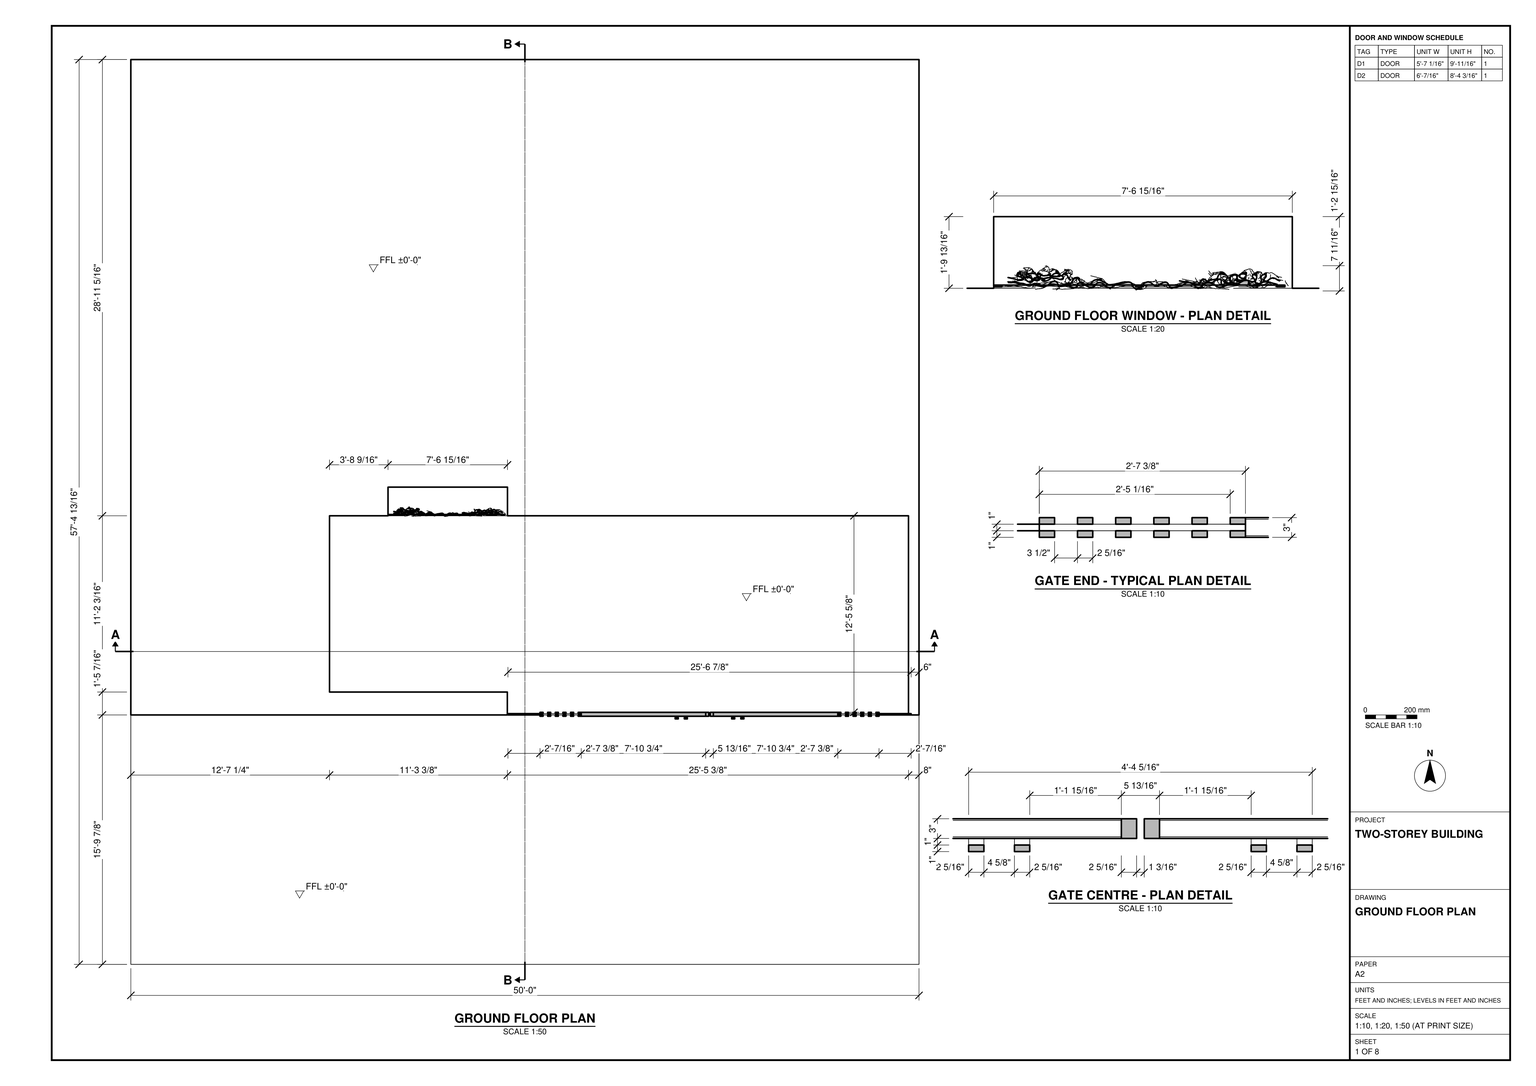
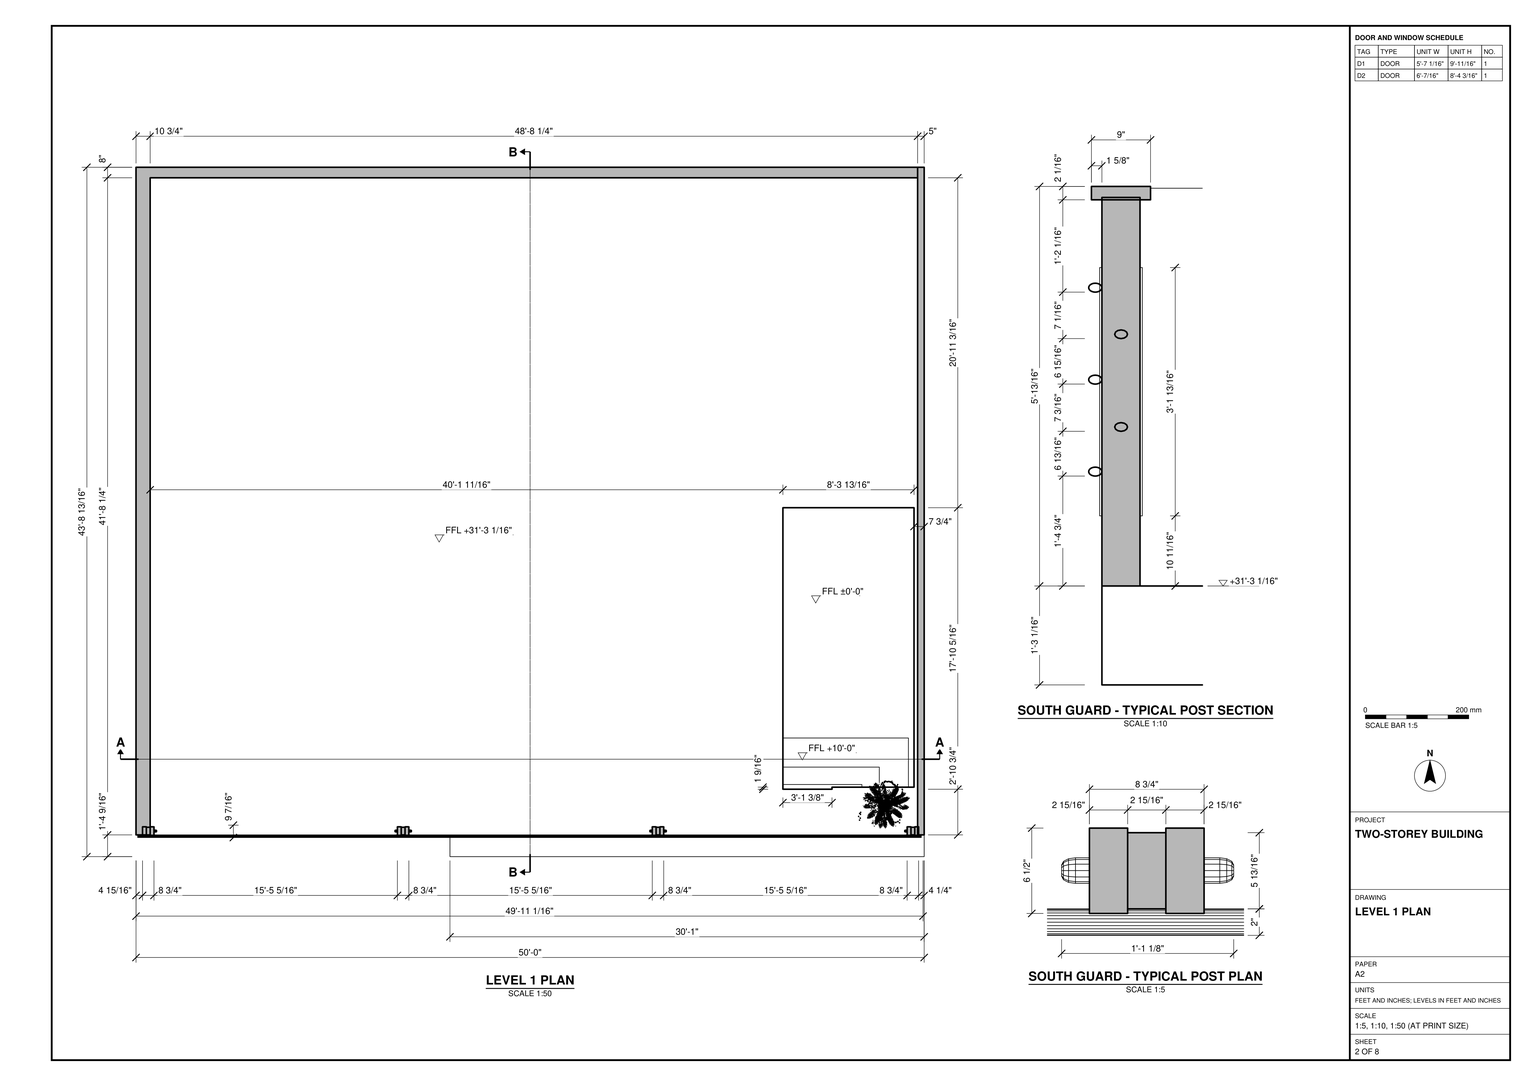
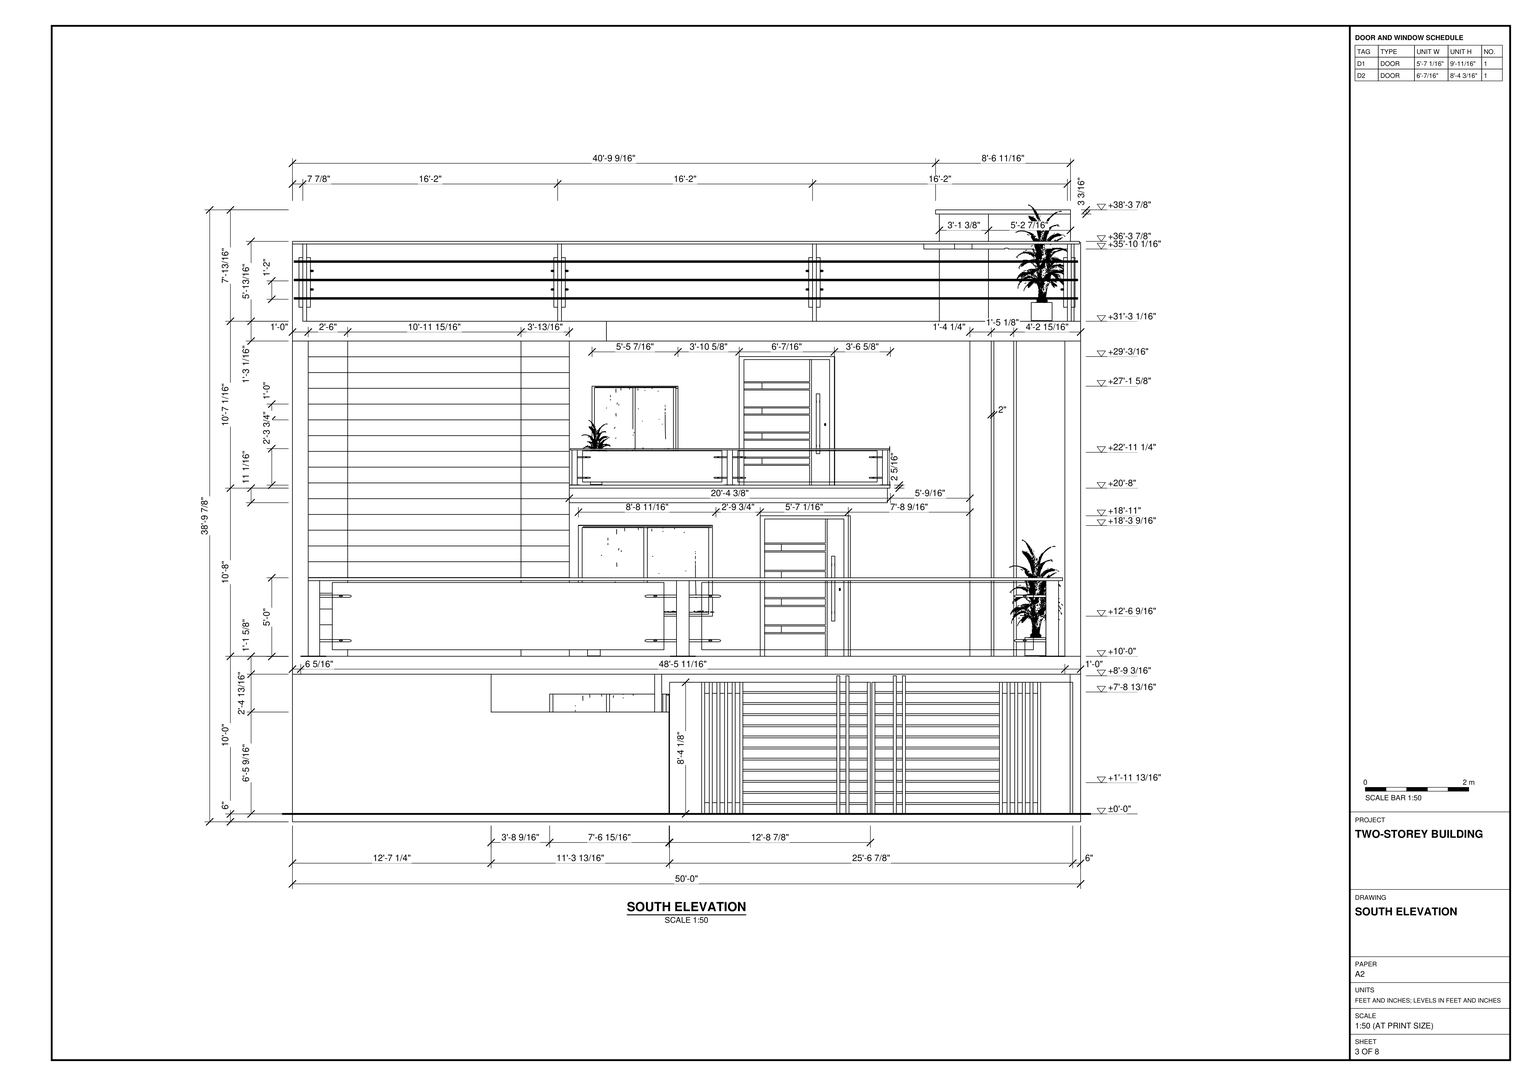
Build the two-storey building in SketchUp from task_files/diagram_01.pdf. Work in feet and inches. Set out the complete model at 50'-0" wide by 57'-4 13/16" deep, with an overall height of 39'-2 5/8". Use ±0'-0" as the ground-floor datum and +31'-3 1/16" as the upper terrace level.

Follow the plans for the ground slab, wall returns, wall thicknesses and projecting ground-floor window feature. On the south frontage, place the two-leaf gate to the right of the stepped solid wall. Use the gate details to distinguish the horizontal slats from the closely spaced vertical end members. Above the gate, model the broad lower balcony and the shorter balcony above it, including their slab edges and panel guards. Set the windows and doors behind the guards as shown in elevation, with the horizontally divided wall panel to their left. Model the flat roof terrace with its rectangular opening, perimeter walls and post-and-rail guard along the south edge.

Keep walls, slabs, roof and each furniture or joinery piece shown in separate groups or components. Use components for repeated parts such as guard posts. Decor and loose items, including plants, may be any suitable library components. Save one SketchUp model as output_files/two_storey_building_with_balconies_and_a_gated_frontage.skp.

# SketchUp Ruby script. Lengths in inches.
U = 1.inch
M = Sketchup.active_model
def pt(a) = Geom::Point3d.new(a.map { |v| v * U })
def face(e, loops, mat)
  f = e.add_face(loops[0].map { |a| pt(a) })
  loops[1..].each { |l| e.add_face(l.map { |a| pt(a) }).erase! }
  f.material = f.back_material = mat if mat
  f
end
# faces: each face lists its corners as indices into pts; further lists are holes
def faces(e, pts, list, mat = nil) = list.each { |f| face(e, (f[0].is_a?(Array) ? f : [f]).map { |l| l.map { |i| pts[i] } }, mat) }
# xy, xz, yz: faces in a plane at the given z, y or x. An outline is a flat list of corners, or four numbers for a rectangle; further outlines are holes
def ring(l) = l.size == 4 ? [[l[0], l[1]], [l[2], l[1]], [l[2], l[3]], [l[0], l[3]]] : l.each_slice(2).to_a
def flat(e, list, mat, &to3) = list.each { |f| face(e, (f[0].is_a?(Array) ? f : [f]).map { |l| ring(l).map { |u, v| to3.(u, v) } }, mat) }
def xy(e, z, list, mat = nil) = flat(e, list, mat) { |x, y| [x, y, z] }
def xz(e, y, list, mat = nil) = flat(e, list, mat) { |x, z| [x, y, z] }
def yz(e, x, list, mat = nil) = flat(e, list, mat) { |y, z| [x, y, z] }
def lines(e, pts, list) = list.each { |a, b| e.add_line(pt(pts[a]), pt(pts[b])) }
# prism: a flat outline (further loops are holes) pulled along v
def prism(e, loops, v, mat = nil)
  f = face(e, loops, mat); d = Geom::Vector3d.new(v.map { |x| x * U })
  f.pushpull(f.normal.samedirection?(d) ? d.length : -d.length)
end
def box(e, o, s, mat = nil) = prism(e, [[o, [o[0] + s[0], o[1], o[2]], [o[0] + s[0], o[1] + s[1], o[2]], [o[0], o[1] + s[1], o[2]]]], [0, 0, s[2]], mat)
def at(x, y, z, deg = 0) = Geom::Transformation.translation(pt([x, y, z])) * Geom::Transformation.rotation(ORIGIN, Z_AXIS, deg.degrees)
def axes(o, x, y, z) = Geom::Transformation.new([*x, 0, *y, 0, *z, 0, *pt(o).to_a, 1])
def part(name) = M.definitions.add(name)
# library, detail: a bought-in or finely detailed component or shape, given as its bounding box
def library(name, o, s) = part(name).tap { |d| box(d.entities, o, s) }
def detail(e, o, s) = box(e.add_group.entities, o, s)
def put(e, d, t, mat = nil) = e.add_instance(d, t).tap { |i| i.material = mat if mat }
def group(e, t, mat = nil) = e.add_group.tap { |g| g.transformation = t; g.material = mat if mat }.entities
root = M.entities
M.materials.add("EWSZ RGF 1").color = [166, 112, 73]
M.materials.add("VBGD1").color = [203, 203, 203]
M.materials.add("W4E SDT G1").color = [255, 255, 255]
M.materials.add("W4E SESF XVD1").color = [203, 203, 203]
M.materials.add("[0131_Silver]").color = [192, 192, 192]
M.materials.add("[Color M07]").color = [58, 58, 58]
M.materials.add("[Color_002]").color = [172, 198, 184]
M.materials["[Color_002]"].alpha = 0.07
M.materials.add("[Field Rectangle Tile]").color = [196, 189, 179]
M.materials.add("[Wood Veneer 01]").color = [120, 70, 37]
c1 = part("Panel mounting bracket")
xy(c1.entities,-0.08,[[2.57,0.63,2.46,0.64,2.36,0.69,2.28,0.75,2.21,0.84,2.17,0.9375,2.15,1.05,2.17,1.15,2.21,1.25,2.27,1.34,2.36,1.41,2.46,1.45,2.57,1.46,2.68,1.45,2.78,1.41,2.86,1.34,2.93,1.26,2.97,1.16,2.99,1.05,2.97,0.94,2.93,0.84,2.87,0.75,2.78,0.6875,2.68,0.64]])
xy(c1.entities,0,[[0.79,0,0.68,0.01,0.58,0.03,0.49,0.06,0.39,0.11,0.31,0.16,0.23,0.23,0.16,0.31,0.11,0.39,0.06,0.49,0.03,0.58,0.01,0.68,0,0.79,0,1.1,0.01,1.21,0.03,1.31,0.06,1.4,0.11,1.5,0.16,1.58,0.23,1.66,0.31,1.73,0.39,1.78,0.49,1.83,0.58,1.86,0.68,1.88,0.79,1.89,7.875,1.89,7.875,0]])
xy(c1.entities,0.2,[[[0.79,0,0.68,0.01,0.58,0.03,0.49,0.06,0.39,0.11,0.31,0.16,0.23,0.23,0.16,0.31,0.11,0.39,0.06,0.49,0.03,0.58,0.01,0.68,0,0.79,0,1.1,0.01,1.21,0.03,1.31,0.06,1.4,0.11,1.5,0.16,1.58,0.23,1.66,0.31,1.73,0.39,1.78,0.49,1.83,0.58,1.86,0.68,1.88,0.79,1.89,7.875,1.89,7.875,0],[2.57,0.63,2.68,0.64,2.78,0.6875,2.87,0.75,2.93,0.84,2.97,0.94,2.99,1.05,2.97,1.16,2.93,1.26,2.86,1.34,2.78,1.41,2.68,1.45,2.57,1.46,2.46,1.45,2.36,1.41,2.27,1.34,2.21,1.25,2.17,1.15,2.15,1.05,2.17,0.9375,2.21,0.84,2.28,0.75,2.36,0.69,2.46,0.64]],[2.57,0.63,2.68,0.64,2.78,0.6875,2.87,0.75,2.93,0.84,2.97,0.94,2.99,1.05,2.97,1.16,2.93,1.26,2.86,1.34,2.78,1.41,2.68,1.45,2.57,1.46,2.46,1.45,2.36,1.41,2.27,1.34,2.21,1.25,2.17,1.15,2.15,1.05,2.17,0.9375,2.21,0.84,2.28,0.75,2.36,0.69,2.46,0.64]])
xy(c1.entities,0.68,[[2.57,0.63,2.46,0.64,2.36,0.69,2.28,0.75,2.21,0.84,2.17,0.9375,2.15,1.05,2.17,1.15,2.21,1.25,2.27,1.34,2.36,1.41,2.46,1.45,2.57,1.46,2.68,1.45,2.78,1.41,2.86,1.34,2.93,1.26,2.97,1.16,2.99,1.05,2.97,0.94,2.93,0.84,2.87,0.75,2.78,0.6875,2.68,0.64]])
xz(c1.entities,0,[[0.79,0,7.875,0.2]])
xz(c1.entities,1.89,[[0.79,0,7.875,0.08],[0.79,0.08,7.875,0.2]])
yz(c1.entities,0,[[0.79,0,1.1,0.08],[0.79,0.08,1.1,0.2]])
p = [[2.46,0.64,-0.08],[2.46,0.64,0.2],[2.36,0.69,0.2],[2.36,0.69,-0.08],[2.57,0.63,-0.08],[2.57,0.63,0.2],
  [2.68,0.64,-0.08],[2.68,0.64,0.2],[2.78,0.6875,-0.08],[2.78,0.6875,0.2],[2.28,0.75,0.2],[2.28,0.75,-0.08],
  [2.87,0.75,-0.08],[2.87,0.75,0.2],[2.21,0.84,-0.08],[2.21,0.84,0.2],[2.17,0.9375,0.2],[2.17,0.9375,-0.08],
  [2.93,0.84,-0.08],[2.93,0.84,0.2],[2.97,0.94,-0.08],[2.97,0.94,0.2],[2.15,1.05,0.2],[2.15,1.05,-0.08],
  [2.99,1.05,-0.08],[2.99,1.05,0.2],[2.17,1.15,0.2],[2.17,1.15,-0.08],[2.97,1.16,-0.08],[2.97,1.16,0.2],
  [2.21,1.25,0.2],[2.21,1.25,-0.08],[2.93,1.26,-0.08],[2.93,1.26,0.2],[2.27,1.34,0.2],[2.27,1.34,-0.08],
  [2.36,1.41,0.2],[2.36,1.41,-0.08],[2.78,1.41,-0.08],[2.78,1.41,0.2],[2.86,1.34,0.2],[2.86,1.34,-0.08],
  [2.46,1.45,0.2],[2.46,1.45,-0.08],[2.68,1.45,-0.08],[2.68,1.45,0.2],[2.57,1.46,0.2],[2.57,1.46,-0.08],
  [0.49,0.06,0.2],[0.49,0.06,0],[0.58,0.03,0],[0.58,0.03,0.2],[0.68,0.01,0],[0.68,0.01,0.2],
  [0.79,0,0],[0.79,0,0.2],[0.31,0.16,0.2],[0.31,0.16,0.08],[0.31,0.16,0],[0.39,0.11,0],
  [0.39,0.11,0.2],[0.23,0.23,0],[0.23,0.23,0.08],[0.16,0.31,0.08],[0.16,0.31,0],[0.11,0.39,0.08],
  [0.11,0.39,0],[0.06,0.49,0.08],[0.06,0.49,0],[0.03,0.58,0.08],[0.03,0.58,0],[0.01,0.68,0.08],
  [0.01,0.68,0],[0,0.79,0.08],[0,0.79,0],[0,1.1,0],[0,1.1,0.08],[0.01,1.21,0.08],
  [0.01,1.21,0],[0.03,1.31,0.08],[0.03,1.31,0],[0.06,1.4,0.08],[0.06,1.4,0],[0.11,1.5,0.08],
  [0.11,1.5,0],[0.16,1.58,0.08],[0.16,1.58,0],[0.23,1.66,0.08],[0.23,1.66,0],[0.31,1.73,0.08],
  [0.31,1.73,0],[0.39,1.78,0.08],[0.39,1.78,0],[0.49,1.83,0.08],[0.49,1.83,0],[0.58,1.86,0.08],
  [0.58,1.86,0],[0.68,1.88,0.08],[0.68,1.88,0],[0.79,1.89,0.08],[0.79,1.89,0],[0.23,0.23,0.2],
  [0.16,0.31,0.2],[0.11,0.39,0.2],[0.06,0.49,0.2],[0.03,0.58,0.2],[0.01,0.68,0.2],[0,0.79,0.2],
  [0,1.1,0.2],[0.01,1.21,0.2],[0.03,1.31,0.2],[0.06,1.4,0.2],[0.11,1.5,0.2],[0.16,1.58,0.2],
  [0.23,1.66,0.2],[0.31,1.73,0.2],[0.39,1.78,0.2],[0.49,1.83,0.2],[0.58,1.86,0.2],[0.68,1.88,0.2],
  [0.79,1.89,0.2],[2.46,0.64,0.68],[2.36,0.69,0.68],[2.57,0.63,0.68],[2.68,0.64,0.68],[2.78,0.6875,0.68],
  [2.28,0.75,0.68],[2.87,0.75,0.68],[2.21,0.84,0.68],[2.17,0.9375,0.68],[2.97,0.94,0.68],[2.93,0.84,0.68],
  [2.15,1.05,0.68],[2.99,1.05,0.68],[2.17,1.15,0.68],[2.97,1.16,0.68],[2.21,1.25,0.68],[2.93,1.26,0.68],
  [2.27,1.34,0.68],[2.36,1.41,0.68],[2.78,1.41,0.68],[2.86,1.34,0.68],[2.46,1.45,0.68],[2.68,1.45,0.68],
  [2.57,1.46,0.68]]
faces(c1.entities,p,[[0,1,2,3],[4,5,1,0],[6,7,5,4],[8,9,7,6],[3,2,10,11],[12,13,9,8],[14,15,16,17],[11,10,15,14],
  [18,19,13,12],[20,21,19,18],[17,16,22,23],[24,25,21,20],[23,22,26,27],[28,29,25,24],[27,26,30,31],[32,33,29,28],
  [31,30,34,35],[35,34,36,37],[38,39,40,41],[41,40,33,32],[37,36,42,43],[44,45,39,38],[43,42,46,47],[47,46,45,44],
  [48,49,50,51],[51,50,52,53],[53,52,54,55],[56,57,58,59,60],[60,59,49,48],[61,62,63,64],[58,57,62,61],[64,63,65,66],
  [66,65,67,68],[68,67,69,70],[70,69,71,72],[72,71,73,74],[75,76,77,78],[78,77,79,80],[80,79,81,82],[82,81,83,84],
  [84,83,85,86],[86,85,87,88],[88,87,89,90],[90,89,91,92],[92,91,93,94],[94,93,95,96],[96,95,97,98],[98,97,99,100],
  [63,62,101,102],[62,57,56,101],[65,63,102,103],[67,65,103,104],[69,67,104,105],[71,69,105,106],[73,71,106,107],[77,76,108,109],
  [79,77,109,110],[81,79,110,111],[83,81,111,112],[85,83,112,113],[87,85,113,114],[89,87,114,115],[91,89,115,116],[93,91,116,117],
  [95,93,117,118],[97,95,118,119],[99,97,119,120],[2,1,121,122],[1,5,123,121],[5,7,124,123],[7,9,125,124],[10,2,122,126],
  [9,13,127,125],[15,10,126,128],[16,15,128,129],[19,21,130,131],[13,19,131,127],[22,16,129,132],[21,25,133,130],[26,22,132,134],
  [25,29,135,133],[30,26,134,136],[29,33,137,135],[34,30,136,138],[36,34,138,139],[40,39,140,141],[33,40,141,137],[42,36,139,142],
  [39,45,143,140],[46,42,142,144],[45,46,144,143]])
c2 = part("Glass balcony railing")
xy(c2.entities,0,[[0,0,3.9375,6.3],[0,92.32,3.9375,98.62],[0,184.64,3.9375,190.9375]])
xy(c2.entities,0.39,[[0,0,3.9375,1.57],[0,1.57,1.18,4.72],[1.18,1.57,1.97,4.72],[1.97,1.57,2.76,4.72],[2.76,1.57,3.9375,4.72],
  [0,4.72,3.9375,6.3],[0,92.32,3.9375,93.89],[0,93.89,1.18,97.04],[1.18,93.89,1.97,97.04],[1.97,93.89,2.76,97.04],
  [2.76,93.89,3.9375,97.04],[0,97.04,3.9375,98.62],[0,184.64,3.9375,186.21],[0,186.21,1.18,189.36],[1.18,186.21,1.97,189.36],
  [1.97,186.21,2.76,189.36],[2.76,186.21,3.9375,189.36],[0,189.36,3.9375,190.9375]])
xy(c2.entities,5.55,[[1.46,7.875,1.85,90.76],[1.46,100.19,1.85,183.08]],"[Color_002]")
xy(c2.entities,60.67,[[1.46,7.875,1.85,90.76]],"[Color_002]")
xy(c2.entities,62.2,[[[0.79,0.57,1.18,0.57,1.18,4.72,2.76,4.72,2.76,0.57,3.15,0.57,3.15,190.36,2.76,190.36,2.76,186.21,1.18,186.21,1.18,190.36,0.79,190.36],[1.18,93.89,2.76,97.04]],[1.18,0.57,1.97,1.57],[1.97,0.57,2.76,1.57],[1.18,1.57,1.97,2.36],[1.97,1.57,2.76,2.36],
  [1.18,2.36,1.57,3.9375],[1.57,2.36,1.97,3.9375],[1.97,2.36,2.36,3.9375],[2.36,2.36,2.76,3.9375],[1.18,3.9375,1.97,4.72],
  [1.97,3.9375,2.76,4.72],[1.18,93.89,1.97,94.68],[1.97,93.89,2.76,94.68],[1.18,94.68,1.57,96.26],[1.57,94.68,1.97,96.26],
  [1.97,94.68,2.36,96.26],[2.36,94.68,2.76,96.26],[1.18,96.26,1.97,97.04],[1.97,96.26,2.76,97.04],[1.18,186.21,1.97,187],
  [1.97,186.21,2.76,187],[1.18,187,1.57,188.58],[1.57,187,1.97,188.58],[1.97,187,2.36,188.58],[2.36,187,2.76,188.58],
  [1.18,188.58,1.97,189.36],[1.97,188.58,2.76,189.36],[1.18,189.36,1.97,190.36],[1.97,189.36,2.76,190.36]])
xy(c2.entities,64.57,[[0.79,0.57,1.97,190.36],[1.97,0.57,3.15,190.36]])
xz(c2.entities,0,[[0,0,3.9375,0.39]])
xz(c2.entities,0.57,[[0.79,62.2,3.15,64.57]])
xz(c2.entities,1.57,[[1.18,0.39,2.76,62.2]])
xz(c2.entities,4.72,[[1.18,0.39,2.76,13.9375],[1.18,13.9375,2.76,50.39],[1.18,50.39,2.76,62.2]])
xz(c2.entities,6.3,[[0,0,3.9375,0.39]])
xz(c2.entities,7.875,[[1.46,5.55,1.85,60.67]],"[Color_002]")
xz(c2.entities,90.76,[[1.46,5.55,1.85,60.67]],"[Color_002]")
xz(c2.entities,92.32,[[0,0,3.9375,0.39]])
xz(c2.entities,93.89,[[1.18,0.39,2.76,62.2]])
xz(c2.entities,97.04,[[1.18,0.39,2.76,13.9375],[1.18,13.9375,2.76,50.39],[1.18,50.39,2.76,62.2]])
xz(c2.entities,98.62,[[0,0,3.9375,0.39]])
xz(c2.entities,183.08,[[1.46,5.55,1.85,60.67]],"[Color_002]")
xz(c2.entities,184.64,[[0,0,3.9375,0.39]])
xz(c2.entities,186.21,[[1.18,0.39,2.76,62.2]])
xz(c2.entities,189.36,[[1.18,0.39,2.76,13.9375],[1.18,13.9375,2.76,50.39],[1.18,50.39,2.76,62.2]])
xz(c2.entities,190.36,[[0.79,62.2,3.15,64.57]])
xz(c2.entities,190.9375,[[0,0,3.9375,0.39]])
yz(c2.entities,0,[[0,0,6.3,0.39],[92.32,0,98.62,0.39],[184.64,0,190.9375,0.39]])
yz(c2.entities,0.79,[[0.57,62.2,190.36,64.57]])
yz(c2.entities,1.18,[[1.57,0.39,4.72,62.2],[93.89,0.39,97.04,62.2],[186.21,0.39,189.36,62.2]])
yz(c2.entities,1.46,[[7.875,5.55,90.76,60.67]],"[Color_002]")
yz(c2.entities,1.85,[[7.875,5.55,90.76,60.67]],"[Color_002]")
yz(c2.entities,2.76,[[1.57,0.39,4.72,62.2],[93.89,0.39,97.04,62.2],[186.21,0.39,189.36,62.2]])
yz(c2.entities,3.15,[[0.57,62.2,190.36,64.57]])
yz(c2.entities,3.9375,[[0,0,6.3,0.39],[92.32,0,98.62,0.39],[184.64,0,190.9375,0.39]])
p = [[1.85,100.19,7.77],[1.85,100.18,7.91],[1.46,100.21,7.61],[1.46,100.19,7.77],[1.46,183.08,60.67],[1.46,100.19,60.67],
  [1.85,100.19,60.67],[1.85,183.08,60.67],[1.85,7.875,58.45],[1.85,7.86,58.31],[1.85,100.19,5.55],[1.46,100.19,5.55]]
lines(c2.entities,p,[[0,1],[2,3],[4,5],[5,3],[0,6],[6,5],[7,6],[8,9],[0,10],[11,2]])
put(c2.entities,c1,axes([2.05,86.02,12.05],[0,1,0],[0,0,1],[-1,0,0]))
put(c2.entities,c1,axes([2.05,12.6,48.5],[0,-1,0],[0,0,1],[-1,0,0]))
put(c2.entities,c1,axes([2.05,12.6,12.05],[0,-1,0],[0,0,1],[-1,0,0]))
put(c2.entities,c1,axes([2.05,178.34,48.5],[0,1,0],[0,0,1],[-1,0,0]))
put(c2.entities,c1,axes([2.05,86.02,48.5],[0,1,0],[0,0,1],[-1,0,0]))
put(c2.entities,c1,axes([2.05,104.92,12.05],[0,-1,0],[0,0,1],[-1,0,0]))
put(c2.entities,c1,axes([2.05,104.92,48.5],[0,-1,0],[0,0,1],[-1,0,0]))
put(c2.entities,c1,axes([2.05,178.34,12.05],[0,1,0],[0,0,1],[-1,0,0]))
c3 = library("Door 3",[97.98,35.29,0],[39.37,9.06,86.61])
c4 = part("Box01")
box(c4.entities,[-154.71,-4.5,86.47],[308.77,9,3],"EWSZ RGF 1")
c5 = part("Box12")
box(c5.entities,[-150.65,-2.9,0],[1.5,5.8,87],"W4E SDT G1")
c6 = part("Box14")
box(c6.entities,[-152.15,-3.25,15.7],[1.5,6.5,55.61],"EWSZ RGF 1")
c7 = part("ChamferCy6")
yz(c7.entities,-153.25,[[0.01,55.94,-0.2,56,-0.36,56.16,-0.41,56.37,-0.36,56.58,-0.2,56.74,0.01,56.8,0.23,56.74,0.39,56.58,0.44,56.37,0.39,56.16,0.23,56]],"W4E SESF XVD1")
yz(c7.entities,-146.49,[[0.01,55.94,0.23,56,0.39,56.16,0.44,56.37,0.39,56.58,0.23,56.74,0.01,56.8,-0.2,56.74,-0.36,56.58,-0.41,56.37,-0.36,56.16,-0.2,56]],"W4E SESF XVD1")
p = [[-152.7,0.01,55.4],[-152.7,-0.47,55.53],[-152.97,-0.4375,55.59],[-152.97,0.01,55.47],[-147.04,0.01,55.4],[-147.04,-0.47,55.53],
  [-146.77,0.01,55.47],[-146.77,-0.4375,55.59],[-152.7,0.5,55.53],[-152.97,0.46,55.59],[-147.04,0.5,55.53],[-146.77,0.46,55.59],
  [-152.7,-0.83,55.88],[-152.97,-0.77,55.92],[-147.04,-0.83,55.88],[-146.77,-0.77,55.92],[-153.17,-0.34,55.76],[-153.17,0.01,55.67],
  [-146.57,0.01,55.67],[-146.57,-0.34,55.76],[-153.17,0.36,55.76],[-146.57,0.36,55.76],[-152.7,0.86,55.88],[-152.97,0.79,55.92],
  [-147.04,0.86,55.88],[-146.77,0.79,55.92],[-153.17,-0.59,56.02],[-146.57,-0.59,56.02],[-153.17,0.62,56.02],[-146.57,0.62,56.02],
  [-153.25,-0.2,56],[-153.25,0.01,55.94],[-146.49,0.01,55.94],[-146.49,-0.2,56],[-153.25,0.23,56],[-146.49,0.23,56],
  [-153.25,-0.36,56.16],[-146.49,-0.36,56.16],[-153.25,0.39,56.16],[-146.49,0.39,56.16],[-152.7,-0.96,56.37],[-152.97,-0.89,56.37],
  [-147.04,-0.96,56.37],[-146.77,-0.89,56.37],[-153.17,-0.6875,56.37],[-146.57,-0.6875,56.37],[-152.97,0.91,56.37],[-153.17,0.72,56.37],
  [-146.57,0.72,56.37],[-146.77,0.91,56.37],[-152.7,0.99,56.37],[-147.04,0.99,56.37],[-153.25,-0.41,56.37],[-146.49,-0.41,56.37],
  [-153.25,0.44,56.37],[-146.49,0.44,56.37],[-152.7,-0.83,56.86],[-152.97,-0.77,56.82],[-147.04,-0.83,56.86],[-146.77,-0.77,56.82],
  [-153.17,-0.59,56.72],[-146.57,-0.59,56.72],[-153.25,-0.36,56.58],[-146.49,-0.36,56.58],[-153.17,0.62,56.72],[-153.25,0.39,56.58],
  [-146.49,0.39,56.58],[-146.57,0.62,56.72],[-152.97,0.79,56.82],[-146.77,0.79,56.82],[-152.7,0.86,56.86],[-147.04,0.86,56.86],
  [-153.17,-0.34,56.98],[-153.25,-0.2,56.74],[-146.49,-0.2,56.74],[-146.57,-0.34,56.98],[-153.17,0.36,56.98],[-153.25,0.23,56.74],
  [-146.49,0.23,56.74],[-146.57,0.36,56.98],[-152.97,-0.4375,57.15],[-146.77,-0.4375,57.15],[-153.17,0.01,57.07],[-153.25,0.01,56.8],
  [-146.49,0.01,56.8],[-146.57,0.01,57.07],[-152.97,0.46,57.15],[-146.77,0.46,57.15],[-152.7,-0.47,57.21],[-147.04,-0.47,57.21],
  [-152.7,0.5,57.21],[-147.04,0.5,57.21],[-152.97,0.01,57.27],[-146.77,0.01,57.27],[-152.7,0.01,57.34],[-147.04,0.01,57.34]]
faces(c7.entities,p,[[0,1,2,3],[4,5,1,0],[6,7,5,4],[8,0,3,9],[10,4,0,8],[11,6,4,10],[1,12,13,2],[5,14,12,1],
  [7,15,14,5],[3,2,16,17],[18,19,7,6],[9,3,17,20],[21,18,6,11],[22,8,9,23],[24,10,8,22],[25,11,10,24],
  [2,13,26,16],[19,27,15,7],[23,9,20,28],[29,21,11,25],[17,16,30,31],[32,33,19,18],[20,17,31,34],[35,32,18,21],
  [16,26,36,30],[33,37,27,19],[28,20,34,38],[39,35,21,29],[12,40,41,13],[14,42,40,12],[15,43,42,14],[13,41,44,26],
  [27,45,43,15],[46,23,28,47],[48,29,25,49],[50,22,23,46],[49,25,24,51],[51,24,22,50],[26,44,52,36],[37,53,45,27],
  [47,28,38,54],[55,39,29,48],[40,56,57,41],[42,58,56,40],[43,59,58,42],[41,57,60,44],[45,61,59,43],[44,60,62,52],
  [53,63,61,45],[64,47,54,65],[66,55,48,67],[68,46,47,64],[67,48,49,69],[70,50,46,68],[69,49,51,71],[71,51,50,70],
  [60,72,73,62],[63,74,75,61],[76,64,65,77],[78,66,67,79],[57,80,72,60],[61,75,81,59],[72,82,83,73],[74,84,85,75],
  [82,76,77,83],[84,78,79,85],[86,68,64,76],[79,67,69,87],[56,88,80,57],[59,81,89,58],[90,70,68,86],[87,69,71,91],
  [58,89,88,56],[91,71,70,90],[80,92,82,72],[75,85,93,81],[92,86,76,82],[85,79,87,93],[88,94,92,80],[89,95,94,88],
  [81,93,95,89],[94,90,86,92],[95,91,90,94],[93,87,91,95]],"W4E SESF XVD1")
c8 = part("Cylinder01")
prism(c8.entities,[[[-154.05,-3.21,67.51],[-154.05,-3.05,67.3],[-154.05,-2.95,67.06],[-154.05,-2.92,66.8],[-154.05,-2.95,66.54],[-154.05,-3.05,66.3],[-154.05,-3.21,66.09],[-154.05,-3.42,65.93],[-154.05,-3.66,65.83],[-154.05,-3.92,65.8],[-154.05,-4.18,65.83],[-154.05,-4.42,65.93],[-154.05,-4.625,66.09],[-154.05,-4.78,66.3],[-154.05,-4.88,66.54],[-154.05,-4.92,66.8],[-154.05,-4.88,67.06],[-154.05,-4.78,67.3],[-154.05,-4.625,67.51],[-154.05,-4.42,67.67],[-154.05,-4.18,67.77],[-154.05,-3.92,67.8],[-154.05,-3.66,67.77],[-154.05,-3.42,67.67]]],[307.45,0,0],"VBGD1")
c9 = part("skp269")
put(c9.entities,c4,at(0,0,0))
put(c9.entities,c5,at(0,0,0))
put(c9.entities,c6,at(0,0,0))
put(c9.entities,c7,at(0,0,0))
put(c9.entities,c8,at(0,0,0))
put(c9.entities,c6,at(3,0,0))
put(c9.entities,c7,at(0,0,-20.76))
put(c9.entities,c8,at(0,0,-20.59))
put(c9.entities,c8,at(0,0,-41.18))
put(c9.entities,c5,at(100,0,0))
put(c9.entities,c6,at(103,0,0))
put(c9.entities,c7,at(100,0,0))
put(c9.entities,c6,at(100,0,0))
put(c9.entities,c7,at(100,0,-20.76))
put(c9.entities,c6,at(200,0,0))
put(c9.entities,c7,at(200,0,-20.76))
put(c9.entities,c7,at(200,0,0))
put(c9.entities,c5,at(200,0,0))
put(c9.entities,c6,at(203,0,0))
put(c9.entities,c5,at(300,0,0))
put(c9.entities,c7,at(300,0,0))
put(c9.entities,c6,at(300,0,0))
put(c9.entities,c7,at(300,0,-20.76))
put(c9.entities,c6,at(303,0,0))
c10 = part("Railing1")
put(c10.entities,c9,at(150.65,2.9,0))
c11 = part("Vertical gate bar")
box(c11.entities,[0,0,0],[1,1,71])
c12 = part("Gate stile")
box(c12.entities,[0,0,0],[1,3,71],"[0131_Silver]")
c13 = part("Slatted gate leaf")
xy(c13.entities,0,[[24,0,64.75,3]])
xy(c13.entities,0,[[0,1,24,2]],"[0131_Silver]")
xy(c13.entities,5,[[24,0,64.75,0.25],[24,2.75,64.75,3]],"[0131_Silver]")
xy(c13.entities,6,[[24,0,64.75,0.25],[10.5,1,24,2],[24,2.75,64.75,3]],"[0131_Silver]")
xy(c13.entities,11,[[24,0,64.75,0.25],[24,2.75,64.75,3]],"[0131_Silver]")
xy(c13.entities,12,[[24,0,64.75,0.25],[24,2.75,64.75,3]],"[0131_Silver]")
xy(c13.entities,17,[[24,0,64.75,0.25],[24,2.75,64.75,3]],"[0131_Silver]")
xy(c13.entities,18,[[24,0,64.75,0.25],[24,2.75,64.75,3]],"[0131_Silver]")
xy(c13.entities,23,[[24,0,64.75,0.25],[24,2.75,64.75,3]],"[0131_Silver]")
xy(c13.entities,24,[[24,0,64.75,0.25],[24,2.75,64.75,3]],"[0131_Silver]")
xy(c13.entities,29,[[24,0,64.75,0.25],[24,2.75,64.75,3]],"[0131_Silver]")
xy(c13.entities,30,[[24,0,64.75,0.25],[24,2.75,64.75,3]],"[0131_Silver]")
xy(c13.entities,35,[[24,0,64.75,0.25],[24,2.75,64.75,3]],"[0131_Silver]")
xy(c13.entities,36,[[24,0,64.75,0.25],[24,2.75,64.75,3]],"[0131_Silver]")
xy(c13.entities,41,[[24,0,64.75,0.25],[24,2.75,64.75,3]],"[0131_Silver]")
xy(c13.entities,42,[[24,0,64.75,0.25],[24,2.75,64.75,3]],"[0131_Silver]")
xy(c13.entities,47,[[24,0,64.75,0.25],[24,2.75,64.75,3]],"[0131_Silver]")
xy(c13.entities,48,[[24,0,64.75,0.25],[24,2.75,64.75,3]],"[0131_Silver]")
xy(c13.entities,53,[[24,0,64.75,0.25],[24,2.75,64.75,3]],"[0131_Silver]")
xy(c13.entities,54,[[24,0,64.75,0.25],[24,2.75,64.75,3]],"[0131_Silver]")
xy(c13.entities,59,[[24,0,64.75,0.25],[24,2.75,64.75,3]],"[0131_Silver]")
xy(c13.entities,60,[[24,0,64.75,0.25],[24,2.75,64.75,3]],"[0131_Silver]")
xy(c13.entities,65,[[10.5,1,24,2]])
xy(c13.entities,65,[[24,0,64.75,0.25],[24,2.75,64.75,3]],"[0131_Silver]")
xy(c13.entities,66,[[24,0,64.75,0.25],[24,2.75,64.75,3]],"[0131_Silver]")
xy(c13.entities,71,[[24,0,64.75,3]])
xy(c13.entities,71,[[0,1,24,2]],"[0131_Silver]")
xz(c13.entities,0,[[24,0,64.75,5],[24,6,64.75,11],[24,12,64.75,17],[24,18,64.75,23],[24,24,64.75,29],
  [24,30,64.75,35],[24,36,64.75,41],[24,42,64.75,47],[24,48,64.75,53],[24,54,64.75,59],
  [24,60,64.75,65],[24,66,64.75,71]])
xz(c13.entities,0.25,[[24,5,64.75,6],[24,11,64.75,12],[24,17,64.75,18],[24,23,64.75,24],[24,29,64.75,30],
  [24,35,64.75,36],[24,41,64.75,42],[24,47,64.75,48],[24,53,64.75,54],[24,59,64.75,60],
  [24,65,64.75,66]],"[0131_Silver]")
xz(c13.entities,1,[[0,0,24,0,24,6,10.5,6,10.5,65,24,65,24,71,0,71]],"[0131_Silver]")
xz(c13.entities,2,[[0,0,0,71,24,71,24,65,10.5,65,10.5,6,24,6,24,0]],"[0131_Silver]")
xz(c13.entities,2.75,[[24,5,64.75,6],[24,11,64.75,12],[24,17,64.75,18],[24,23,64.75,24],[24,29,64.75,30],
  [24,35,64.75,36],[24,41,64.75,42],[24,47,64.75,48],[24,53,64.75,54],[24,59,64.75,60],
  [24,65,64.75,66]],"[0131_Silver]")
xz(c13.entities,3,[[24,0,64.75,5],[24,6,64.75,11],[24,12,64.75,17],[24,18,64.75,23],[24,24,64.75,29],
  [24,30,64.75,35],[24,36,64.75,41],[24,42,64.75,47],[24,48,64.75,53],[24,54,64.75,59],
  [24,60,64.75,65],[24,66,64.75,71]])
yz(c13.entities,0,[[1,0,2,71]],"[0131_Silver]")
yz(c13.entities,10.5,[[1,6,2,65]],"[0131_Silver]")
yz(c13.entities,24,[[0,0,1,5],[1,0,2,6],[2,0,2,6,2.75,6,2.75,5,3,5,3,0],[0.25,5,0.25,6,0,6,0,11,0.25,11,0.25,12,0,12,0,17,0.25,17,0.25,18,0,18,0,23,0.25,23,0.25,24,0,24,0,29,0.25,29,0.25,30,0,30,0,35,0.25,35,0.25,36,0,36,0,41,0.25,41,0.25,42,0,42,0,47,0.25,47,0.25,48,0,48,0,53,0.25,53,0.25,54,0,54,0,59,0.25,59,0.25,60,0,60,0,65,3,65,3,60,2.75,60,2.75,59,3,59,3,54,2.75,54,2.75,53,3,53,3,48,2.75,48,2.75,47,3,47,3,42,2.75,42,2.75,41,3,41,3,36,2.75,36,2.75,35,3,35,3,30,2.75,30,2.75,29,3,29,3,24,2.75,24,2.75,23,3,23,3,18,2.75,18,2.75,17,3,17,3,12,2.75,12,2.75,11,3,11,3,6,1,6,1,5],[0.25,65,0.25,66,0,66,0,71,1,71,1,65],
  [1,65,2,71],[2,65,2,71,3,71,3,66,2.75,66,2.75,65]])
yz(c13.entities,64.75,[[0,0,3,0,3,5,2.75,5,2.75,6,3,6,3,11,2.75,11,2.75,12,3,12,3,17,2.75,17,2.75,18,3,18,3,23,2.75,23,2.75,24,3,24,3,29,2.75,29,2.75,30,3,30,3,35,2.75,35,2.75,36,3,36,3,41,2.75,41,2.75,42,3,42,3,47,2.75,47,2.75,48,3,48,3,53,2.75,53,2.75,54,3,54,3,59,2.75,59,2.75,60,3,60,3,65,2.75,65,2.75,66,3,66,3,71,0,71,0,66,0.25,66,0.25,65,0,65,0,60,0.25,60,0.25,59,0,59,0,54,0.25,54,0.25,53,0,53,0,48,0.25,48,0.25,47,0,47,0,42,0.25,42,0.25,41,0,41,0,36,0.25,36,0.25,35,0,35,0,30,0.25,30,0.25,29,0,29,0,24,0.25,24,0.25,23,0,23,0,18,0.25,18,0.25,17,0,17,0,12,0.25,12,0.25,11,0,11,0,6,0.25,6,0.25,5,0,5]])
put(c13.entities,c11,at(10.5,0,0),"[0131_Silver]")
put(c13.entities,c11,at(10.5,2,0),"[0131_Silver]")
put(c13.entities,c11,at(13,2,0),"[0131_Silver]")
put(c13.entities,c11,at(13,0,0),"[0131_Silver]")
put(c13.entities,c11,at(15.5,0,0),"[0131_Silver]")
put(c13.entities,c11,at(18,0,0),"[0131_Silver]")
put(c13.entities,c11,at(20.5,0,0),"[0131_Silver]")
put(c13.entities,c12,at(64.75,0,0),"[0131_Silver]")
put(c13.entities,c11,at(23,0,0),"[0131_Silver]")
put(c13.entities,c11,at(15.5,2,0),"[0131_Silver]")
put(c13.entities,c11,at(18,2,0),"[0131_Silver]")
put(c13.entities,c11,at(20.5,2,0),"[0131_Silver]")
put(c13.entities,c11,at(23,2,0),"[0131_Silver]")
c14 = part("Gate frame upright")
prism(c14.entities,[[[0,1,0],[0,0,0],[0,0,2.5],[0,-2,2.5],[0,-2,-70.3125],[0,-1,-70.3125],[0,-1,-71.3125],[0,-3,-71.3125],[0,-3,3.5],[0,1,3.5]]],[1,0,0])
c15 = part("Double entrance gate")
put(c15.entities,c13,at(0,2,0.3125))
put(c15.entities,c13,axes([132,2,0.3125],[-1,0,0],[0,1,0],[0,0,1]))
put(c15.entities,c14,at(57.75,3,71.3125),"[0131_Silver]")
put(c15.entities,c14,at(54.75,3,71.3125),"[0131_Silver]")
put(c15.entities,c14,at(73.25,3,71.3125),"[0131_Silver]")
put(c15.entities,c14,at(76.25,3,71.3125),"[0131_Silver]")
c16 = part("gate")
put(c16.entities,c15,at(133.6875,221.625,-0.3125))
c17 = library("plant",[-22.43,-22.29,0],[44.86,44.58,89.56])
c18 = library("Group\#4",[0,0,0],[98.51,23.72,124.8])
xy(root,-6,[[0,0,600,688.8125]])
xy(root,0,[[0,0,600,0,600,189.875,592,189.875,592,341.5,151.25,341.5,151.25,207.31,286.62,207.31,286.62,189.875,0,189.875],[0,189.875,286.62,189.875,286.62,207.31,151.25,207.31,151.25,341.5,592,341.5,592,189.875,600,189.875,600,688.8125,0,688.8125]])
xy(root,23.81,[[195.79,341.5,286.72,363.3125]])
xy(root,77.5625,[[[151.25,189.875,286.62,207.31],[278.41,196.7,277.71,196.79,277.0625,197.06,276.51,197.49,276.08,198.04,275.8125,198.69,275.72,199.39,275.8125,200.08,276.08,200.73,276.51,201.29,277.0625,201.72,277.71,201.98,278.41,202.08,279.1,201.98,279.75,201.72,280.31,201.29,280.74,200.73,281,200.08,281.1,199.39,281,198.69,280.74,198.04,280.31,197.49,279.75,197.06,279.1,196.79]]])
xy(root,91.24,[[195.79,341.5,286.72,363.3125]])
xy(root,106.375,[[0,180.5625,151.25,189.875],[[151.25,180.5625,151.25,341.5,592,341.5,592,189.875,600,189.875,600,180.5625],[278.41,196.7,279.1,196.79,279.75,197.06,280.31,197.49,280.74,198.04,281,198.69,281.1,199.39,281,200.08,280.74,200.73,280.31,201.29,279.75,201.72,279.1,201.98,278.41,202.08,277.71,201.98,277.0625,201.72,276.51,201.29,276.08,200.73,275.8125,200.08,275.72,199.39,275.8125,198.69,276.08,198.04,276.51,197.49,277.0625,197.06,277.71,196.79]]])
xy(root,120,[[12,180.5625,588,180.5625,588,254.3125,424.72,254.3125,424.72,281.1875,356.1,281.1875,356.1,254.3125,210.77,254.3125,210.77,222.625,12,222.625]])
xy(root,150.54,[[217.66,254.3125,319.6,348.8125]])
xy(root,219.79,[[217.66,254.3125,319.6,348.8125]])
xy(root,227,[[356.1,254.3125,424.72,281.1875]])
xy(root,236.9375,[[210.77,222.625,452.92,254.3125]])
xy(root,248,[[210.77,216.4375,210.77,222.625,452.92,222.625,452.92,254.3125,454.8,254.3125,454.8,216.4375],[210.77,222.625,210.77,224.625,449.55,224.625,449.55,254.3125,452.92,254.3125,452.92,222.625],[210.77,224.625,449.55,224.625,449.55,254.3125,412.82,254.3125,412.82,275.25,340.07,275.25,340.07,254.3125,210.77,254.3125]])
xy(root,250.3125,[[210.77,216.4375,454.8,216.4375,454.8,254.3125,449.55,254.3125,449.55,224.625,210.77,224.625]])
xy(root,275.27,[[228.04,254.3125,293.48,285.4375]])
xy(root,325.64,[[228.04,254.3125,293.48,285.4375]])
xy(root,348.1875,[[340.07,254.3125,412.82,275.25]])
xy(root,360,[[[239,164,239,180.5625,210.77,180.5625,210.77,254.3125,588,254.3125,588,164],[261.15,186.15,565.85,186.15,565.85,232.16,232.92,232.16,232.92,202.72,261.15,202.72]],[0,180.5625,0,688.8125,600,688.8125,600,180.5625,588,180.5625,588,254.3125,210.77,254.3125,210.77,222.625,12,222.625,12,180.5625],[12,180.5625,210.77,222.625],[[261.15,186.15,261.15,202.72,232.92,202.72,232.92,232.16,565.85,232.16,565.85,186.15],[274.4,199.4,552.6,199.4,552.6,218.91,246.17,218.91,246.17,215.96,274.4,215.96]],[274.4,199.4,274.4,215.96,246.17,215.96,246.17,218.91,552.6,218.91,552.6,199.4]])
xy(root,360,[[588,164,600,180.5625]],"[Color M07]")
xy(root,375.0625,[[239,164,600,180.5625],[[10.78,180.5625,595,680.8125],[492.46,215.33,492.46,429.64,592.27,429.64,592.27,216.89,529.83,216.89,529.83,215.33]],[595,180.5625,600,688.8125]])
xy(root,430.0625,[[480.64,203.33,480.64,217.33,492.46,217.33,492.46,215.33,504.06,215.33,504.06,203.33],[517.34,203.33,517.34,215.33,529.83,215.33,529.83,216.89,542.31,216.89,542.31,203.33],[544.88,203.33,567.29,216.89],[570.35,203.33,592.27,216.89],[504.06,215.33,517.34,216.89],
  [480.64,217.33,492.46,267.72],[480.64,270.41,492.46,320.8],[480.64,323.48,492.46,373.875],[480.64,376.5625,492.46,429.64]])
xy(root,430.75,[[542.31,203.33,544.88,216.89]])
xy(root,431.25,[[567.29,203.33,570.35,216.89]])
xy(root,435.0625,[[595,180.5625,600,688.8125],[480.64,203.33,504.06,203.33,504.06,216.01,492.46,216.01,492.46,267.72,480.64,267.72],[517.34,203.33,592.27,203.33,592.27,216.89,529.83,216.89,529.83,216.01,517.34,216.01],[492.46,216.01,492.46,429.64,592.27,429.64,592.27,216.89,529.83,216.89,529.83,216.01,517.34,216.01,517.34,216.89,504.06,216.89,504.06,216.01],[504.06,216.01,517.34,216.89],
  [480.64,267.72,492.46,270.41],[480.64,270.41,492.46,320.8],[480.64,320.8,492.46,323.48],[480.64,323.48,492.46,373.875],[480.64,373.875,492.46,376.5625],
  [480.64,376.5625,492.46,429.64],[10.78,680.8125,595,688.8125]])
xy(root,435.625,[[0,180.5625,10.78,688.8125]])
xy(root,456.6875,[[489.58,215.08,489.58,429.64,492.46,429.64,492.46,216.01,529.83,216.01,529.83,216.89,592.27,216.89,592.27,215.08],[492.46,216.01,492.46,429.64,592.27,429.64,592.27,216.89,529.83,216.89,529.83,216.01]])
xy(root,459.875,[[489.58,215.08,592.27,429.64]])
xz(root,0,[[0,-6,600,0]])
xz(root,164,[[239,360,600,375.0625]],"[Color M07]")
xz(root,180.5625,[[595,375.0625,600,435.0625]])
xz(root,180.5625,[[0,106.375,600,106.375,600,120,12,120,12,360,0,360],[588,120,600,360],[0,360,239,360,239,375.0625,10.78,375.0625,10.78,435.625,0,435.625]],"[Color M07]")
xz(root,189.875,[[0,0,286.62,0,286.62,77.5625,151.25,77.5625,151.25,106.375,0,106.375],[592,0,600,106.375]])
xz(root,203.33,[[480.64,430.0625,504.06,435.0625],[517.34,430.0625,542.31,430.0625,542.31,430.75,544.88,430.75,544.88,430.0625,567.29,430.0625,567.29,431.25,570.35,431.25,570.35,430.0625,592.27,430.0625,592.27,435.0625,517.34,435.0625]])
xz(root,207.31,[[151.25,0,286.62,77.5625]])
xz(root,215.08,[[489.58,456.6875,592.27,459.875]])
xz(root,215.33,[[492.46,375.0625,529.83,430.0625]])
xz(root,216.01,[[492.46,435.0625,529.83,456.6875]])
xz(root,216.4375,[[210.77,248,454.8,250.3125]])
xz(root,216.89,[[504.06,430.0625,517.34,435.0625]])
xz(root,216.89,[[529.83,375.0625,592.27,375.0625,592.27,430.0625,570.35,430.0625,570.35,431.25,567.29,431.25,567.29,430.0625,544.88,430.0625,544.88,430.75,542.31,430.75,542.31,430.0625,529.83,430.0625],[529.83,435.0625,592.27,456.6875]],"[Field Rectangle Tile]")
xz(root,222.625,[[210.77,236.9375,452.92,248]])
xz(root,222.625,[[12,120,42.03,132],[42.03,120,173.98,132],[173.98,120,210.77,132],[12,132,42.03,144],[42.03,132,173.98,144],
  [173.98,132,210.77,144],[12,144,42.03,156],[42.03,144,173.98,156],[173.98,144,210.77,156],[12,156,42.03,168],
  [42.03,156,173.98,168],[173.98,156,210.77,168],[12,168,42.03,180],[42.03,168,173.98,180],[173.98,168,210.77,180],
  [12,180,42.03,192],[42.03,180,173.98,192],[173.98,180,210.77,192],[12,192,42.03,204],[42.03,192,173.98,204],
  [173.98,192,210.77,204],[12,204,42.03,216],[42.03,204,173.98,216],[173.98,204,210.77,216],[12,216,42.03,228],
  [42.03,216,173.98,228],[173.98,216,210.77,228],[12,228,42.03,240],[42.03,228,173.98,240],[173.98,228,210.77,240],
  [12,240,42.03,252],[42.03,240,173.98,252],[173.98,240,210.77,252],[12,252,42.03,264],[42.03,252,173.98,264],
  [173.98,252,210.77,264],[12,264,42.03,276],[42.03,264,173.98,276],[173.98,264,210.77,276],[12,276,42.03,288],
  [42.03,276,173.98,288],[173.98,276,210.77,288],[12,288,42.03,300],[42.03,288,173.98,300],[173.98,288,210.77,300],
  [12,300,42.03,312],[42.03,300,173.98,312],[173.98,300,210.77,312],[12,312,42.03,324],[42.03,312,173.98,324],
  [173.98,312,210.77,324],[12,324,42.03,336],[42.03,324,173.98,336],[173.98,324,210.77,336],[12,336,42.03,348],
  [42.03,336,173.98,348],[173.98,336,210.77,348],[12,348,42.03,360],[42.03,348,173.98,360],[173.98,348,210.77,360]],"[Wood Veneer 01]")
xz(root,224.625,[[210.77,248,449.55,250.3125]])
xz(root,254.3125,[[[210.77,120,356.1,120,356.1,227,424.72,227,424.72,120,515.7,120,515.7,360,210.77,360,210.77,248,340.07,248,340.07,348.1875,412.82,348.1875,412.82,248,449.55,248,449.55,250.3125,454.8,250.3125,454.8,248,452.92,248,452.92,236.9375,210.77,236.9375],[217.66,150.54,319.6,219.79],[228.04,275.27,293.48,325.64]],[531.95,120,533.95,360],[549.08,120,551.08,360],[449.55,248,452.92,250.3125],[452.92,248,453.05,250.3125],
  [453.05,248,454.8,250.3125]])
xz(root,254.3125,[[515.7,120,531.95,360],[533.95,120,549.08,360],[551.08,120,588,360]],"[Field Rectangle Tile]")
xz(root,267.72,[[480.64,430.0625,492.46,435.0625]])
xz(root,270.41,[[480.64,430.0625,492.46,435.0625]])
xz(root,275.25,[[340.07,248,412.82,348.1875]])
xz(root,281.1875,[[356.1,120,424.72,227]])
xz(root,285.4375,[[228.04,275.27,293.48,325.64]])
xz(root,320.8,[[480.64,430.0625,492.46,435.0625]])
xz(root,323.48,[[480.64,430.0625,492.46,435.0625]])
xz(root,341.5,[[[151.25,0,592,106.375],[195.79,23.81,286.72,91.24]]])
xz(root,348.8125,[[217.66,150.54,319.6,219.79]])
xz(root,363.3125,[[195.79,23.81,286.72,91.24]])
xz(root,373.875,[[480.64,430.0625,492.46,435.0625]])
xz(root,376.5625,[[480.64,430.0625,492.46,435.0625]])
xz(root,429.64,[[492.46,375.0625,492.46,430.0625,480.64,430.0625,480.64,435.0625,592.27,435.0625,592.27,375.0625],[492.46,435.0625,592.27,456.6875],[489.58,456.6875,592.27,459.875]])
xz(root,680.8125,[[10.78,375.0625,595,435.0625]])
xz(root,688.8125,[[0,-6,600,0],[0,0,600,120],[0,120,600,240],[0,240,600,360],[0,360,0,435.625,10.78,435.625,10.78,435.0625,595,435.0625,595,375.0625,600,375.0625,600,360],
  [595,375.0625,600,435.0625]])
yz(root,0,[[0,-6,688.8125,0],[189.875,0,189.875,106.375,180.5625,106.375,180.5625,120,688.8125,120,688.8125,0],[180.5625,120,688.8125,240],[180.5625,240,688.8125,360],[180.5625,360,688.8125,435.625]])
yz(root,10.78,[[180.5625,375.0625,680.8125,375.0625,680.8125,435.0625,688.8125,435.0625,688.8125,435.625,180.5625,435.625]])
yz(root,12,[[180.5625,120,222.625,360]])
yz(root,151.25,[[207.31,0,341.5,0,341.5,106.375,189.875,106.375,189.875,77.5625,207.31,77.5625]])
yz(root,195.79,[[341.5,23.81,363.3125,91.24]])
yz(root,210.77,[[222.625,120,254.3125,236.9375],[216.4375,248,222.625,250.3125],[222.625,248,224.625,250.3125],[224.625,248,254.3125,248,254.3125,360,222.625,360,222.625,250.3125,224.625,250.3125]])
yz(root,217.66,[[254.3125,150.54,348.8125,219.79]])
yz(root,228.04,[[254.3125,275.27,285.4375,325.64]])
yz(root,239,[[164,360,180.5625,375.0625]],"[Color M07]")
yz(root,286.62,[[189.875,0,207.31,77.5625]])
yz(root,286.72,[[341.5,23.81,363.3125,91.24]])
yz(root,293.48,[[254.3125,275.27,285.4375,325.64]])
yz(root,319.6,[[254.3125,150.54,348.8125,219.79]])
yz(root,340.07,[[254.3125,248,275.25,348.1875]])
yz(root,356.1,[[254.3125,120,281.1875,227]])
yz(root,412.82,[[254.3125,248,275.25,348.1875]])
yz(root,424.72,[[254.3125,120,281.1875,227]])
yz(root,449.55,[[224.625,248,254.3125,250.3125]])
yz(root,452.92,[[222.625,236.9375,254.3125,248]])
yz(root,454.8,[[216.4375,248,254.3125,250.3125]])
yz(root,480.64,[[203.33,430.0625,267.72,435.0625],[270.41,430.0625,320.8,435.0625],[323.48,430.0625,373.875,435.0625],[376.5625,430.0625,429.64,435.0625]])
yz(root,489.58,[[215.08,456.6875,429.64,459.875]])
yz(root,492.46,[[215.33,375.0625,215.33,430.0625,267.72,430.0625,267.72,435.0625,270.41,435.0625,270.41,430.0625,320.8,430.0625,320.8,435.0625,323.48,435.0625,323.48,430.0625,373.875,430.0625,373.875,435.0625,376.5625,435.0625,376.5625,430.0625,429.64,430.0625,429.64,375.0625],[216.01,435.0625,429.64,456.6875]])
yz(root,504.06,[[203.33,430.0625,216.89,435.0625]])
yz(root,517.34,[[203.33,430.0625,216.89,435.0625]])
yz(root,529.83,[[215.33,375.0625,216.89,430.0625],[216.01,435.0625,216.89,456.6875]])
yz(root,542.31,[[203.33,430.0625,216.89,430.75]])
yz(root,544.88,[[203.33,430.0625,216.89,430.75]])
yz(root,567.29,[[203.33,430.0625,216.89,431.25]])
yz(root,570.35,[[203.33,430.0625,216.89,431.25]])
yz(root,588,[[180.5625,120,254.3125,360]],"[Field Rectangle Tile]")
yz(root,592,[[189.875,0,341.5,106.375]])
yz(root,592.27,[[216.89,375.0625,429.64,375.0625,429.64,435.0625,203.33,435.0625,203.33,430.0625,216.89,430.0625],[216.89,435.0625,429.64,456.6875],[215.08,456.6875,429.64,459.875]])
yz(root,595,[[180.5625,375.0625,680.8125,435.0625],[680.8125,375.0625,688.8125,435.0625]])
yz(root,600,[[0,-6,688.8125,0],[189.875,0,688.8125,0,688.8125,360,180.5625,360,180.5625,106.375,189.875,106.375],[164,360,688.8125,375.0625],[180.5625,375.0625,688.8125,435.0625]])
p = [[277.71,196.79,77.5625],[278.41,196.7,77.5625],[278.41,196.7,106.375],[277.71,196.79,106.375],[279.1,196.79,77.5625],[279.1,196.79,106.375],
  [277.0625,197.06,77.5625],[277.0625,197.06,106.375],[279.75,197.06,77.5625],[279.75,197.06,106.375],[276.51,197.49,77.5625],[276.51,197.49,106.375],
  [280.31,197.49,77.5625],[280.31,197.49,106.375],[276.08,198.04,77.5625],[276.08,198.04,106.375],[280.74,198.04,77.5625],[280.74,198.04,106.375],
  [275.8125,198.69,77.5625],[275.8125,198.69,106.375],[281,198.69,77.5625],[281,198.69,106.375],[275.72,199.39,77.5625],[275.72,199.39,106.375],
  [281.1,199.39,77.5625],[281.1,199.39,106.375],[275.8125,200.08,77.5625],[275.8125,200.08,106.375],[281,200.08,77.5625],[281,200.08,106.375],
  [276.08,200.73,77.5625],[276.08,200.73,106.375],[280.74,200.73,77.5625],[280.74,200.73,106.375],[276.51,201.29,77.5625],[276.51,201.29,106.375],
  [280.31,201.29,77.5625],[280.31,201.29,106.375],[277.0625,201.72,77.5625],[277.0625,201.72,106.375],[279.75,201.72,77.5625],[279.75,201.72,106.375],
  [277.71,201.98,77.5625],[277.71,201.98,106.375],[279.1,201.98,77.5625],[279.1,201.98,106.375],[278.41,202.08,77.5625],[278.41,202.08,106.375]]
faces(root,p,[[0,1,2,3],[1,4,5,2],[6,0,3,7],[4,8,9,5],[10,6,7,11],[8,12,13,9],[14,10,11,15],[12,16,17,13],
  [18,14,15,19],[16,20,21,17],[22,18,19,23],[20,24,25,21],[26,22,23,27],[24,28,29,25],[30,26,27,31],[28,32,33,29],
  [34,30,31,35],[32,36,37,33],[38,34,35,39],[36,40,41,37],[42,38,39,43],[40,44,45,41],[46,42,43,47],[44,46,47,45]])
put(root,c2,axes([454.52,216.4375,250.3125],[0.0714,0,0],[0,0.19836,0],[0,0,0.45471]))
put(root,c2,axes([210.77,226.5625,250.3125],[0,-1,0],[1.28,0,0],[0,0,0.43]))
put(root,c3,axes([159.78,219.02,248],[1.84,0,0],[0,1,0],[0,0,1.15671]))
put(root,c3,axes([189.22,219.02,118.34],[1.70311,0,0],[0,1,0],[0,0,1.25454]))
put(root,c2,axes([6.33,184.5,119.83],[0,-1,0],[3.0464,0,0],[0,0,0.9288]))
put(root,c10,axes([7.87,180.5625,375.0625],[1.94024,0,0],[0,1,0],[0,0,0.68]))
put(root,c16,axes([-23.75,-34.75,0.13],[2.325,0,0],[0,1,0],[0,0,1.41]))
put(root,c17,axes([229.54,240.72,120],[0.61,0,0],[0,0.61,0],[0,0,0.61]))
put(root,c17,at(565.57,239.73,120))
put(root,c17,axes([231.27,234.99,250.48],[0.5546,0,0],[0,0.5546,0],[0,0,0.5546]))
put(root,c17,at(570.42,202.85,375.06))
put(root,c18,axes([228.06,254.3125,275.27],[0.6641,0,0],[0,0.29,0],[0,0,0.40364]))
put(root,c18,axes([217.68,252.62,150.54],[1.06256,0,0],[0,0.29,0],[0,0,0.55298]))
put(root,c18,axes([195.79,340.67,23.81],[0.92314,0,0],[0,0.3248,0],[0,0,0.55298]))
